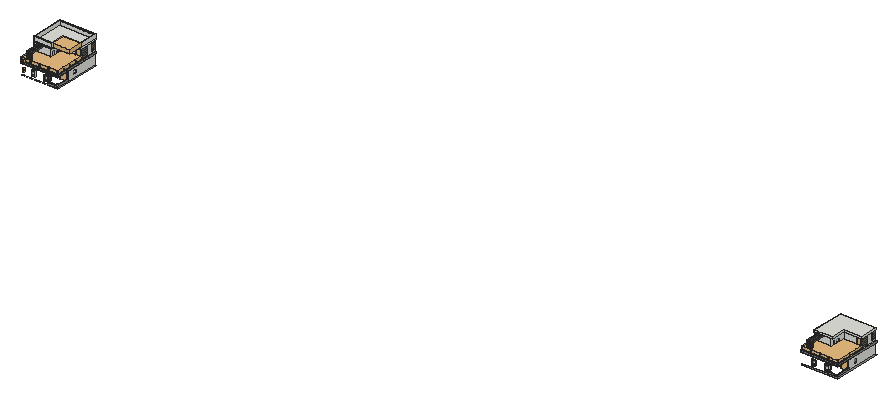
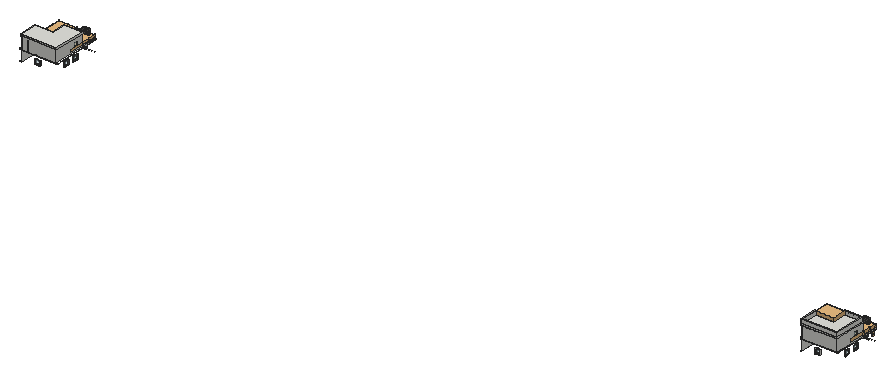
# SketchUp Ruby script. Lengths in inches.
U = 1.inch
M = Sketchup.active_model
def pt(a) = Geom::Point3d.new(a.map { |v| v * U })
def face(e, loops, mat)
  f = e.add_face(loops[0].map { |a| pt(a) })
  loops[1..].each { |l| e.add_face(l.map { |a| pt(a) }).erase! }
  f.material = f.back_material = mat if mat
  f
end
# faces: each face lists its corners as indices into pts; further lists are holes
def faces(e, pts, list, mat = nil) = list.each { |f| face(e, (f[0].is_a?(Array) ? f : [f]).map { |l| l.map { |i| pts[i] } }, mat) }
# xy, xz, yz: faces in a plane at the given z, y or x. An outline is a flat list of corners, or four numbers for a rectangle; further outlines are holes
def ring(l) = l.size == 4 ? [[l[0], l[1]], [l[2], l[1]], [l[2], l[3]], [l[0], l[3]]] : l.each_slice(2).to_a
def flat(e, list, mat, &to3) = list.each { |f| face(e, (f[0].is_a?(Array) ? f : [f]).map { |l| ring(l).map { |u, v| to3.(u, v) } }, mat) }
def xy(e, z, list, mat = nil) = flat(e, list, mat) { |x, y| [x, y, z] }
def xz(e, y, list, mat = nil) = flat(e, list, mat) { |x, z| [x, y, z] }
def yz(e, x, list, mat = nil) = flat(e, list, mat) { |y, z| [x, y, z] }
def lines(e, pts, list) = list.each { |a, b| e.add_line(pt(pts[a]), pt(pts[b])) }
# prism: a flat outline (further loops are holes) pulled along v
def prism(e, loops, v, mat = nil)
  f = face(e, loops, mat); d = Geom::Vector3d.new(v.map { |x| x * U })
  f.pushpull(f.normal.samedirection?(d) ? d.length : -d.length)
end
def box(e, o, s, mat = nil) = prism(e, [[o, [o[0] + s[0], o[1], o[2]], [o[0] + s[0], o[1] + s[1], o[2]], [o[0], o[1] + s[1], o[2]]]], [0, 0, s[2]], mat)
def at(x, y, z, deg = 0) = Geom::Transformation.translation(pt([x, y, z])) * Geom::Transformation.rotation(ORIGIN, Z_AXIS, deg.degrees)
def axes(o, x, y, z) = Geom::Transformation.new([*x, 0, *y, 0, *z, 0, *pt(o).to_a, 1])
def part(name) = M.definitions.add(name)
# library, detail: a bought-in or finely detailed component or shape, given as its bounding box
def library(name, o, s) = part(name).tap { |d| box(d.entities, o, s) }
def detail(e, o, s) = box(e.add_group.entities, o, s)
def put(e, d, t, mat = nil) = e.add_instance(d, t).tap { |i| i.material = mat if mat }
def group(e, t, mat = nil) = e.add_group.tap { |g| g.transformation = t; g.material = mat if mat }.entities
root = M.entities
M.materials.add("Stone C 250cm").color = [107, 104, 102]
M.materials.add("Stone G 100cm").color = [112, 105, 93]
M.materials.add("T8500 Silicone plaster D1 27.81cm").color = [255, 255, 255]
M.materials.add("Wall Paint Bumpy 01 Gray 100cm").color = [135, 135, 135]
M.materials.add("Wood 021 27.52cm").color = [255, 255, 255]
M.materials.add("[Color M06]").color = [86, 86, 86]
M.materials.add("[Translucent Glass Gray]1").color = [128, 128, 128]
M.materials["[Translucent Glass Gray]1"].alpha = 0.5
M.materials.add("[Translucent Glass Safety]").color = [204, 235, 244]
M.materials["[Translucent Glass Safety]"].alpha = 0.5
M.materials.add("[Translucent_Glass_Gray]").color = [128, 128, 128]
M.materials["[Translucent_Glass_Gray]"].alpha = 0.5
c1 = library("Window 46-47",[-61.02,-2.17,0],[122.04,4.34,74.02])
c2 = library("Potted Plant 50-23",[-3.4,-3.5,0],[6.8,7,9.93])
c3 = part("Group\#3")
xy(c3.entities,0,[[0,0,0.83,48],[0.83,0,2.5625,48]])
xy(c3.entities,3,[[0,3,0.67,45],[1.8,3,2.5625,45]])
xy(c3.entities,4.625,[[0.67,4.625,1.8,43.375]])
xy(c3.entities,43.375,[[0.67,4.625,1.8,43.375]])
xy(c3.entities,45,[[0,3,0.67,45],[1.8,3,2.5625,45]])
xy(c3.entities,48,[[0,0,0.83,48],[0.83,0,2.5625,48]])
xz(c3.entities,0,[[0,0,0.83,48],[0.83,0,2.5625,48]])
xz(c3.entities,3,[[0,3,0.67,45],[1.8,3,2.5625,45]])
xz(c3.entities,4.625,[[0.67,4.625,1.8,43.375]])
xz(c3.entities,43.375,[[0.67,4.625,1.8,43.375]])
xz(c3.entities,45,[[0,3,0.67,45],[1.8,3,2.5625,45]])
xz(c3.entities,48,[[0,0,0.83,48],[0.83,0,2.5625,48]])
yz(c3.entities,0,[[[0,0,48,48],[3,3,45,45]]])
yz(c3.entities,0.67,[[[3,3,45,45],[4.625,4.625,43.375,43.375]]])
yz(c3.entities,1.8,[[[3,3,45,45],[4.625,4.625,43.375,43.375]]])
yz(c3.entities,2.5625,[[[0,0,48,48],[3,3,45,45]]])
p = [[1.33,43.375,43.05],[1.33,43.375,4.66],[1.23,4.625,4.66],[1.23,4.625,43.05]]
faces(c3.entities,p,[[0,1,2,3]],"[Translucent Glass Safety]")
c4 = library("Spot Light",[-5.1,-5.1,-11.05],[10.2,10.2,11.05])
c5 = library("Lamp Wall Outdoor 94-02",[-1.89,-4.65,-3.17],[3.78,4.65,6.35])
c6 = part("Group\#7")
p = [[0,43.31,5.11],[2.95,43.31,0],[2.95,0,0],[0,0,5.11]]
faces(c6.entities,p,[[0,1,2,3]],"[Translucent_Glass_Gray]")
c7 = part("Vwntilation window")
put(c7.entities,c6,at(43.48,1.97,32.29))
put(c7.entities,c6,at(43.48,1.97,26.38))
put(c7.entities,c6,at(43.48,1.97,20.48))
put(c7.entities,c6,at(43.48,1.97,14.57))
put(c7.entities,c6,at(43.48,1.97,8.67))
put(c7.entities,c6,at(43.48,1.97,2.76))
g1 = group(c7.entities,at(43.48,0,0))
prism(g1,[[[1.97,47.24,39.37],[1.97,0,39.37],[1.97,0,0],[1.97,47.24,0]],[[1.97,45.28,1.97],[1.97,1.97,1.97],[1.97,1.97,37.4],[1.97,45.28,37.4]]],[-1.97,0,0])
c8 = library("Sphere Light\#7",[-3,-3,-3],[6,6,6])
c9 = library("Sphere Light\#6",[-3,-3,-3],[6,6,6])
c10 = library("Sphere Light\#5",[-3,-3,-3],[6,6,6])
c11 = library("Sphere Light\#8",[-3,-3,-3],[6,6,6])
c12 = library("Door 243 065",[-19.36,-2.49,0],[38.72,4.98,81.96])
c13 = part("Post and beam")
xy(c13.entities,-97.98,[[0,-127.9375,5.5,-124.375]])
xy(c13.entities,0,[[0,-124.375,5.5,0]])
xy(c13.entities,5.4375,[[0,-127.9375,5.5,0]],"Stone C 250cm")
xz(c13.entities,-127.9375,[[0,-97.98,5.5,5.4375]],"Stone C 250cm")
xz(c13.entities,-124.375,[[0,-97.98,5.5,0]])
xz(c13.entities,0,[[0,0,5.5,5.4375]])
yz(c13.entities,0,[[-127.9375,-97.98,-127.9375,5.4375,0,5.4375,0,0,-124.375,0,-124.375,-97.98]],"Stone C 250cm")
yz(c13.entities,5.5,[[-127.9375,-97.98,-124.375,-97.98,-124.375,0,0,0,0,5.4375,-127.9375,5.4375]],"Stone C 250cm")
c14 = part("Group\#6")
xy(c14.entities,0,[[162,13.5,171,46.5],[110.84,153,146.84,162],[298.5,219,331.5,223.5]])
xy(c14.entities,36,[[0,57,9,105],[162,57,171,105]])
xy(c14.entities,84,[[162,13.5,171,46.5],[0,57,9,105],[162,57,171,105],[110.84,153,146.84,162],[298.5,219,331.5,223.5]])
xy(c14.entities,120,[[[0,0,171,0,171,153,351,153,351,328.5,0,328.5],[9,162,9,319.5,342,319.5,342,223.5,294,223.5,294,319.5,289.5,319.5,289.5,219,342,219,342,162],[9,9,162,153]]])
xz(c14.entities,0,[[0,0,171,120]])
xz(c14.entities,9,[[9,0,162,120]])
xz(c14.entities,13.5,[[162,0,171,84]])
xz(c14.entities,46.5,[[162,0,171,84]])
xz(c14.entities,57,[[0,36,9,84],[162,36,171,84]])
xz(c14.entities,105,[[0,36,9,84],[162,36,171,84]])
xz(c14.entities,153,[[9,0,110.84,0,110.84,84,146.84,84,146.84,0,162,0,162,120,9,120],[171,0,351,120]])
xz(c14.entities,162,[[9,0,9,120,342,120,342,0,146.84,0,146.84,84,110.84,84,110.84,0]])
xz(c14.entities,219,[[289.5,0,298.5,0,298.5,84,331.5,84,331.5,0,342,0,342,120,289.5,120]])
xz(c14.entities,223.5,[[294,0,294,120,342,120,342,0,331.5,0,331.5,84,298.5,84,298.5,0]])
xz(c14.entities,319.5,[[9,0,289.5,120],[289.5,0,294,120],[294,0,342,120]])
xz(c14.entities,328.5,[[0,0,351,120]])
yz(c14.entities,0,[[[0,0,328.5,120],[57,36,105,84]]])
yz(c14.entities,9,[[[9,0,153,120],[57,36,105,84]],[162,0,319.5,120]])
yz(c14.entities,110.84,[[153,0,162,84]])
yz(c14.entities,146.84,[[153,0,162,84]])
yz(c14.entities,162,[[[9,0,9,120,153,120,153,0,46.5,0,46.5,84,13.5,84,13.5,0],[57,36,105,84]]])
yz(c14.entities,171,[[[0,0,13.5,0,13.5,84,46.5,84,46.5,0,153,0,153,120,0,120],[57,36,105,84]]])
yz(c14.entities,289.5,[[219,0,319.5,120]])
yz(c14.entities,294,[[223.5,0,319.5,120]])
yz(c14.entities,298.5,[[219,0,223.5,84]])
yz(c14.entities,331.5,[[219,0,223.5,84]])
yz(c14.entities,342,[[162,0,219,120],[223.5,0,319.5,120]])
yz(c14.entities,351,[[153,0,328.5,120]])
c15 = part("Group\#14")
xy(c15.entities,0,[[0,0,2.375,70.51]])
xy(c15.entities,0.3125,[[1.875,0,2.375,70.51]])
xy(c15.entities,0.63,[[1.875,0,2.375,70.51]])
xy(c15.entities,17.3,[[1.875,0,2.375,70.51]])
xy(c15.entities,17.62,[[1.875,0,2.375,70.51]])
xy(c15.entities,34.29,[[1.875,0,2.375,70.51]])
xy(c15.entities,34.61,[[1.875,0,2.375,70.51]])
xy(c15.entities,51.28,[[1.875,0,2.375,70.51]])
xy(c15.entities,51.6,[[1.875,0,2.375,70.51]])
xy(c15.entities,68.28,[[1.875,0,2.375,70.51]])
xy(c15.entities,68.59,[[1.875,0,2.375,70.51]])
xy(c15.entities,85.27,[[1.875,0,2.375,70.51]])
xy(c15.entities,85.58,[[1.875,0,2.375,70.51]],"Stone G 100cm")
xy(c15.entities,102.26,[[1.875,0,2.375,70.51]])
xy(c15.entities,102.57,[[1.875,0,2.375,70.51]])
xy(c15.entities,119.25,[[1.875,0,2.375,70.51]])
xy(c15.entities,119.5625,[[1.875,0,2.375,70.51]],"Stone G 100cm")
xy(c15.entities,120,[[0,0,2.375,70.51]])
xz(c15.entities,0,[[0,0,2.375,0.3125],[0,0.3125,1.875,0.63],[0,17.3,1.875,17.62],[0,34.29,1.875,34.61],[0,51.28,1.875,51.6],
  [0,68.28,1.875,68.59],[0,85.27,1.875,85.58],[0,102.26,1.875,102.57],[0,119.25,1.875,119.5625],[0,119.5625,2.375,120]])
xz(c15.entities,0,[[0,0.63,2.375,17.3],[0,17.62,2.375,34.29],[0,34.61,2.375,51.28],[0,51.6,2.375,68.28],[0,68.59,2.375,85.27],
  [0,85.58,2.375,102.26],[0,102.57,2.375,119.25]],"Stone G 100cm")
xz(c15.entities,70.51,[[0,102.26,1.875,102.57]])
xz(c15.entities,70.51,[[0,0,2.375,0.3125],[0,0.3125,1.875,0.63],[0,0.63,2.375,17.3],[0,17.3,1.875,17.62],[0,17.62,2.375,34.29],
  [0,34.29,1.875,34.61],[0,34.61,2.375,51.28],[0,51.28,1.875,51.6],[0,51.6,2.375,68.28],[0,68.28,1.875,68.59],
  [0,68.59,2.375,85.27],[0,85.27,1.875,85.58],[0,85.58,2.375,102.26],[0,102.57,2.375,119.25],[0,119.25,1.875,119.5625],
  [0,119.5625,2.375,120]],"Stone G 100cm")
yz(c15.entities,0,[[0,0,70.51,120]])
yz(c15.entities,1.875,[[0,119.25,70.51,119.5625]])
yz(c15.entities,1.875,[[0,0.3125,70.51,0.63],[0,17.3,70.51,17.62],[0,34.29,70.51,34.61],[0,51.28,70.51,51.6],[0,68.28,70.51,68.59],
  [0,85.27,70.51,85.58],[0,102.26,70.51,102.57]],"Stone G 100cm")
yz(c15.entities,2.375,[[0,0,70.51,0.3125],[0,0.63,70.51,17.3],[0,17.62,70.51,34.29],[0,34.61,70.51,51.28],[0,51.6,70.51,68.28],
  [0,68.59,70.51,85.27],[0,85.58,70.51,102.26],[0,102.57,70.51,119.25],[0,119.5625,70.51,120]],"Stone G 100cm")
c16 = library("Group\#16",[0,0,0],[44.53,1,120])
c17 = library("Potted Plant 02",[-16.98,-19.78,0],[30.04,38.68,37.52])
c18 = library("Group61\#1",[7976.64,457.72,288.35],[367.58,308.29,25.19])
c19 = library("Ploe",[7975.85,611.43,276.75],[3.15,3.15,37.57])
c20 = part("Group60\#1")
put(c20.entities,c19,at(0,0,0))
put(c20.entities,c19,at(0,-77.25,0))
put(c20.entities,c19,at(0,-154.5,0))
put(c20.entities,c19,at(91.5,-154.5,0))
put(c20.entities,c19,at(183,-154.5,0))
put(c20.entities,c19,at(274.5,-154.5,0))
put(c20.entities,c19,at(366,-154.5,0))
put(c20.entities,c19,at(366,-77.625,0))
put(c20.entities,c19,at(366,-0.75,0))
put(c20.entities,c19,at(366,76.125,0))
put(c20.entities,c19,at(366,153,0))
c21 = part("Group\#11")
put(c21.entities,c18,at(-7975.85,-456.93,-276.75))
put(c21.entities,c20,at(-7975.85,-456.93,-276.75))
c22 = part("Group\#15")
prism(c22.entities,[[[0,0,109.9375],[0,0,0],[2.375,0,0],[2.375,0,0.5],[0.75,0,0.5],[0.75,0,1.5],[2.375,0,1.5],[2.375,0,21.99],[0.75,0,21.99],[0.75,0,22.99],[2.375,0,22.99],[2.375,0,43.48],[0.75,0,43.48],[0.75,0,44.48],[2.375,0,44.48],[2.375,0,64.96],[0.75,0,64.96],[0.75,0,65.96],[2.375,0,65.96],[2.375,0,86.45],[0.75,0,86.45],[0.75,0,87.45],[2.375,0,87.45],[2.375,0,107.9375],[0.75,0,107.9375],[0.75,0,108.9375],[2.375,0,108.9375],[2.375,0,109.9375]]],[0,39.5,0],"Stone G 100cm")
c23 = library("Sphere Light\#4",[-2,-2,-2],[4,4,4])
c24 = library("Sphere Light",[-2,-2,-2],[4,4,4])
c25 = library("Sphere Light\#3",[-2,-2,-2],[4,4,4])
c26 = library("Sphere Light\#2",[-2,-2,-2],[4,4,4])
c27 = library("Sphere Light\#1",[-2,-2,-2],[4,4,4])
c28 = library("Group\#21",[0,0,0],[182.86,140.18,36.98])
xy(root,144.75,[[686.23,450.625,758.23,459.625],[8453.94,661.9,8525.94,670.9]])
xy(root,152.75,[[420.73,290.125,786.73,290.125,786.73,779.125,771.73,779.125,771.73,302.125,475.97,302.125,475.97,293.5625,420.73,293.5625],[8188.44,501.4,8554.44,501.4,8554.44,990.4,8539.44,990.4,8539.44,513.4,8243.6875,513.4,8243.6875,504.84,8188.44,504.84]],"Wall Paint Bumpy 01 Gray 100cm")
xy(root,169.375,[[681.73,302.125,681.73,311.125,762.73,311.125,762.73,450.625,771.73,450.625,771.73,302.125],[8449.44,513.4,8449.44,522.4,8530.44,522.4,8530.44,661.9,8539.44,661.9,8539.44,513.4]])
xy(root,170.375,[[681.73,302.125,771.73,302.125,771.73,450.625,762.73,450.625,762.73,311.125,681.73,311.125],[8449.44,513.4,8539.44,513.4,8539.44,661.9,8530.44,661.9,8530.44,522.4,8449.44,522.4]],"T8500 Silicone plaster D1 27.81cm")
xy(root,176.75,[[512.01,302.125,548.01,311.125],[641.23,302.125,681.73,302.125,681.73,335.125,681.13,335.125,681.13,304.97,641.23,304.97],[641.23,306.1,680.01,306.1,680.01,335.125,679.48,335.125,679.48,306.625,641.23,306.625],[641.23,306.625,679.48,306.625,679.48,335.125,677.23,335.125,677.23,311.125,641.23,311.125],[420.73,507.625,429.73,555.625],
  [762.73,507.625,771.73,555.625],[8279.73,513.4,8315.73,522.4],[8408.94,513.4,8449.44,513.4,8449.44,546.4,8448.85,546.4,8448.85,516.25,8408.94,516.25],[8408.94,517.375,8447.72,517.375,8447.72,546.4,8447.19,546.4,8447.19,517.9,8408.94,517.9],[8408.94,517.9,8447.19,517.9,8447.19,546.4,8444.94,546.4,8444.94,522.4,8408.94,522.4],
  [420.73,618.96,429.73,666.96],[8188.44,718.9,8197.44,766.9],[8530.44,718.9,8539.44,766.9],[590.04,770.125,638.04,779.125],[8188.44,830.24,8197.44,878.24],
  [8357.75,981.4,8405.75,990.4]])
xy(root,178.125,[[642.6,304.97,681.13,304.97,681.13,333.75,680.88,333.75,680.88,305.22,642.6,305.22],[642.6,305.79,680.32,305.79,680.32,333.75,680.01,333.75,680.01,306.1,642.6,306.1],[8410.32,516.25,8448.85,516.25,8448.85,545.03,8448.6,545.03,8448.6,516.5,8410.32,516.5],[8410.32,517.07,8448.03,517.07,8448.03,545.03,8447.72,545.03,8447.72,517.375,8410.32,517.375]])
xy(root,178.8125,[[643.29,305.22,680.88,305.22,680.88,333.0625,680.32,333.0625,680.32,305.79,643.29,305.79],[8411.01,516.5,8448.6,516.5,8448.6,544.34,8448.03,544.34,8448.03,517.07,8411.01,517.07]])
xy(root,222.6875,[[643.29,305.22,643.29,305.79,680.32,305.79,680.32,333.0625,680.88,333.0625,680.88,305.22],[8411.01,516.5,8411.01,517.07,8448.03,517.07,8448.03,544.34,8448.6,544.34,8448.6,516.5]])
xy(root,223.375,[[642.6,304.97,642.6,305.22,680.88,305.22,680.88,333.75,681.13,333.75,681.13,304.97],[642.6,305.79,642.6,306.1,680.01,306.1,680.01,333.75,680.32,333.75,680.32,305.79],[8410.32,516.25,8410.32,516.5,8448.6,516.5,8448.6,545.03,8448.85,545.03,8448.85,516.25],[8410.32,517.07,8410.32,517.375,8447.72,517.375,8447.72,545.03,8448.03,545.03,8448.03,517.07]])
xy(root,224.75,[[512.01,302.125,548.01,311.125],[641.23,302.125,641.23,304.97,681.13,304.97,681.13,335.125,681.73,335.125,681.73,302.125],[641.23,306.1,641.23,306.625,679.48,306.625,679.48,335.125,680.01,335.125,680.01,306.1],[641.23,306.625,641.23,311.125,677.23,311.125,677.23,335.125,679.48,335.125,679.48,306.625],[452.23,360.625,485.23,365.125],
  [633.73,455.125,672.73,459.625],[420.73,507.625,429.73,555.625],[762.73,507.625,771.73,555.625],[8279.73,513.4,8315.73,522.4],[8408.94,513.4,8408.94,516.25,8448.85,516.25,8448.85,546.4,8449.44,546.4,8449.44,513.4],
  [8408.94,517.375,8408.94,517.9,8447.19,517.9,8447.19,546.4,8447.72,546.4,8447.72,517.375],[8408.94,517.9,8408.94,522.4,8444.94,522.4,8444.94,546.4,8447.19,546.4,8447.19,517.9],[8219.94,571.9,8252.94,576.4],[594.73,603.625,633.73,608.125],[420.73,618.96,429.73,666.96],
  [8401.44,666.4,8440.44,670.9],[671.23,680.125,704.23,684.625],[8188.44,718.9,8197.44,766.9],[8530.44,718.9,8539.44,766.9],[590.04,770.125,638.04,779.125],
  [8362.44,814.9,8401.44,819.4],[8188.44,830.24,8197.44,878.24],[8438.94,891.4,8471.94,895.9],[8357.75,981.4,8405.75,990.4]])
xy(root,230.75,[[420.73,387.69,429.73,411.65],[8188.44,598.97,8197.44,622.93],[762.73,691.19,771.73,715.15],[8530.44,902.47,8539.44,926.43]])
xy(root,240.75,[[686.23,450.625,758.23,459.625],[8453.94,661.9,8525.94,670.9]])
xy(root,248.75,[[420.73,387.69,429.73,411.65],[8188.44,598.97,8197.44,622.93],[645.73,644.125,650.23,680.125],[762.73,691.19,771.73,715.15],[8413.44,855.4,8417.94,891.4],
  [8530.44,902.47,8539.44,926.43]])
xy(root,259.75,[[681.73,325.25,681.73,450.25,733.17,450.25,726.6,325.25],[726.6,325.25,733.17,450.25,771.48,450.25,771.48,325.25]])
xy(root,260.75,[[420.73,302.125,681.73,302.125,681.73,450.625,762.73,450.625,762.73,459.625,429.73,459.625,429.73,455.125,489.73,455.125,489.73,365.125,429.73,365.125,429.73,360.625,494.23,360.625,494.23,455.125,677.23,455.125,677.23,311.125,429.73,311.125,429.73,770.125,762.73,770.125,762.73,450.625,771.73,450.625,771.73,779.125,420.73,779.125],[8188.44,513.4,8449.44,513.4,8449.44,661.9,8530.44,661.9,8530.44,670.9,8197.44,670.9,8197.44,666.4,8257.44,666.4,8257.44,576.4,8197.44,576.4,8197.44,571.9,8261.94,571.9,8261.94,666.4,8444.94,666.4,8444.94,522.4,8197.44,522.4,8197.44,981.4,8530.44,981.4,8530.44,661.9,8539.44,661.9,8539.44,990.4,8188.44,990.4],[429.73,603.625,762.73,603.625,762.73,608.125,650.23,608.125,650.23,680.125,762.73,680.125,762.73,684.625,650.23,684.625,650.23,770.125,645.73,770.125,645.73,608.125,429.73,608.125],[8197.44,814.9,8530.44,814.9,8530.44,819.4,8417.94,819.4,8417.94,891.4,8530.44,891.4,8530.44,895.9,8417.94,895.9,8417.94,981.4,8413.44,981.4,8413.44,819.4,8197.44,819.4]])
xy(root,260.75,[[681.73,325.25,771.48,450.25]],"Wood 021 27.52cm")
xy(root,264.75,[[408.73,290.125,408.73,450.625,420.73,450.625,420.73,302.125,774.73,302.125,774.73,775.5,771.73,775.5,771.73,779.125,786.73,779.125,786.73,290.125],[8176.44,501.4,8176.44,661.9,8188.44,661.9,8188.44,513.4,8542.44,513.4,8542.44,986.78,8539.44,986.78,8539.44,990.4,8554.44,990.4,8554.44,501.4]])
xy(root,276.75,[[408.73,290.125,786.73,290.125,786.73,779.125,771.73,779.125,771.73,775.5,774.73,775.5,774.73,302.125,420.73,302.125,420.73,450.625,408.73,450.625],[8176.44,501.4,8554.44,501.4,8554.44,990.4,8539.44,990.4,8539.44,986.78,8542.44,986.78,8542.44,513.4,8188.44,513.4,8188.44,661.9,8176.44,661.9]])
xy(root,401.1875,[[432.73,457.625,594.73,457.625,594.73,600.625,774.73,600.625,774.73,767.125,432.73,767.125],[594.73,457.625,606.73,457.625,606.73,588.89,774.73,588.89,774.73,588.625,786.73,588.625,786.73,595.11,774.73,595.11,774.73,600.625,594.73,600.625]])
xy(root,438.17,[[420.73,445.625,606.73,457.625],[420.73,457.625,432.73,457.625,432.73,767.125,774.73,767.125,774.73,595.11,786.73,595.11,786.73,779.125,420.73,779.125]])
xz(root,290.125,[[408.73,264.75,786.73,276.75]],"Wall Paint Bumpy 01 Gray 100cm")
xz(root,302.125,[[420.73,264.75,774.73,276.75]])
xz(root,302.125,[[681.73,169.375,771.73,170.375]],"T8500 Silicone plaster D1 27.81cm")
xz(root,302.125,[[681.73,152.75,771.73,169.375]],"Wall Paint Bumpy 01 Gray 100cm")
xz(root,304.97,[[641.23,176.75,681.13,176.75,681.13,178.125,642.6,178.125,642.6,223.375,681.13,223.375,681.13,224.75,641.23,224.75]])
xz(root,305.22,[[642.6,178.125,680.88,178.125,680.88,178.8125,643.29,178.8125,643.29,222.6875,680.88,222.6875,680.88,223.375,642.6,223.375]])
xz(root,305.22,[[643.29,178.8125,680.88,222.6875]],"[Translucent Glass Gray]1")
xz(root,305.79,[[642.6,178.125,642.6,223.375,680.32,223.375,680.32,222.6875,643.29,222.6875,643.29,178.8125,680.32,178.8125,680.32,178.125]])
xz(root,306.1,[[641.23,176.75,641.23,224.75,680.01,224.75,680.01,223.375,642.6,223.375,642.6,178.125,680.01,178.125,680.01,176.75]])
xz(root,311.125,[[681.73,169.375,762.73,170.375]])
xz(root,325.25,[[681.73,259.75,771.48,260.75]],"Wood 021 27.52cm")
xz(root,333.0625,[[680.32,178.8125,680.88,222.6875]])
xz(root,333.75,[[680.01,178.125,680.32,223.375],[680.88,178.125,681.13,223.375]])
xz(root,335.125,[[677.23,176.75,679.48,224.75],[679.48,176.75,680.01,224.75],[681.13,176.75,681.73,224.75]])
xz(root,387.69,[[420.73,230.75,429.73,248.75]])
xz(root,411.65,[[420.73,230.75,429.73,248.75]])
xz(root,445.625,[[420.73,401.1875,606.73,438.17]])
xz(root,450.25,[[681.73,259.75,771.48,260.75]])
xz(root,450.625,[[762.73,169.375,771.73,170.375],[762.73,170.375,771.73,260.75],[408.73,264.75,420.73,276.75]])
xz(root,457.625,[[432.73,401.1875,594.73,438.17],[594.73,401.1875,606.73,438.17]])
xz(root,501.4,[[8176.44,264.75,8554.44,276.75]],"Wall Paint Bumpy 01 Gray 100cm")
xz(root,507.625,[[420.73,176.75,429.73,224.75],[762.73,176.75,771.73,224.75]])
xz(root,513.4,[[8188.44,264.75,8542.44,276.75]])
xz(root,513.4,[[8449.44,169.375,8539.44,170.375]],"T8500 Silicone plaster D1 27.81cm")
xz(root,513.4,[[8449.44,152.75,8539.44,169.375]],"Wall Paint Bumpy 01 Gray 100cm")
xz(root,516.25,[[8408.94,176.75,8448.85,176.75,8448.85,178.125,8410.32,178.125,8410.32,223.375,8448.85,223.375,8448.85,224.75,8408.94,224.75]])
xz(root,516.5,[[8410.32,178.125,8448.6,178.125,8448.6,178.8125,8411.01,178.8125,8411.01,222.6875,8448.6,222.6875,8448.6,223.375,8410.32,223.375]])
xz(root,516.5,[[8411.01,178.8125,8448.6,222.6875]],"[Translucent Glass Gray]1")
xz(root,517.07,[[8410.32,178.125,8410.32,223.375,8448.03,223.375,8448.03,222.6875,8411.01,222.6875,8411.01,178.8125,8448.03,178.8125,8448.03,178.125]])
xz(root,517.375,[[8408.94,176.75,8408.94,224.75,8447.72,224.75,8447.72,223.375,8410.32,223.375,8410.32,178.125,8447.72,178.125,8447.72,176.75]])
xz(root,522.4,[[8449.44,169.375,8530.44,170.375]])
xz(root,544.34,[[8448.03,178.8125,8448.6,222.6875]])
xz(root,545.03,[[8447.72,178.125,8448.03,223.375],[8448.6,178.125,8448.85,223.375]])
xz(root,546.4,[[8444.94,176.75,8447.19,224.75],[8447.19,176.75,8447.72,224.75],[8448.85,176.75,8449.44,224.75]])
xz(root,555.625,[[420.73,176.75,429.73,224.75],[762.73,176.75,771.73,224.75]])
xz(root,595.11,[[774.73,401.1875,786.73,438.17]])
xz(root,598.97,[[8188.44,230.75,8197.44,248.75]])
xz(root,618.96,[[420.73,176.75,429.73,224.75]])
xz(root,622.93,[[8188.44,230.75,8197.44,248.75]])
xz(root,661.9,[[8530.44,169.375,8539.44,170.375],[8530.44,170.375,8539.44,260.75],[8176.44,264.75,8188.44,276.75]])
xz(root,666.96,[[420.73,176.75,429.73,224.75]])
xz(root,691.19,[[762.73,230.75,771.73,248.75]])
xz(root,715.15,[[762.73,230.75,771.73,248.75]])
xz(root,718.9,[[8188.44,176.75,8197.44,224.75],[8530.44,176.75,8539.44,224.75]])
xz(root,766.9,[[8188.44,176.75,8197.44,224.75],[8530.44,176.75,8539.44,224.75]])
xz(root,767.125,[[432.73,401.1875,774.73,438.17]])
xz(root,775.5,[[771.73,264.75,774.73,276.75]])
xz(root,779.125,[[771.73,264.75,786.73,276.75],[420.73,401.1875,786.73,438.17]])
xz(root,830.24,[[8188.44,176.75,8197.44,224.75]])
xz(root,878.24,[[8188.44,176.75,8197.44,224.75]])
xz(root,902.47,[[8530.44,230.75,8539.44,248.75]])
xz(root,926.43,[[8530.44,230.75,8539.44,248.75]])
xz(root,986.78,[[8539.44,264.75,8542.44,276.75]])
xz(root,990.4,[[8539.44,264.75,8554.44,276.75]])
yz(root,408.73,[[290.125,264.75,450.625,276.75]])
yz(root,420.73,[[302.125,264.75,450.625,276.75],[445.625,401.1875,457.625,438.17],[457.625,401.1875,779.125,438.17]])
yz(root,432.73,[[457.625,401.1875,767.125,438.17]])
yz(root,512.01,[[302.125,176.75,311.125,224.75]])
yz(root,548.01,[[302.125,176.75,311.125,224.75]])
yz(root,590.04,[[770.125,176.75,779.125,224.75]])
yz(root,606.73,[[445.625,401.1875,457.625,438.17]])
yz(root,638.04,[[770.125,176.75,779.125,224.75]])
yz(root,641.23,[[302.125,176.75,304.97,224.75],[306.1,176.75,306.625,224.75],[306.625,176.75,311.125,224.75]])
yz(root,642.6,[[304.97,178.125,305.22,223.375],[305.79,178.125,306.1,223.375]])
yz(root,643.29,[[305.22,178.8125,305.79,222.6875]])
yz(root,680.01,[[306.1,176.75,306.1,178.125,333.75,178.125,333.75,223.375,306.1,223.375,306.1,224.75,335.125,224.75,335.125,176.75]])
yz(root,680.32,[[305.79,178.125,305.79,178.8125,333.0625,178.8125,333.0625,222.6875,305.79,222.6875,305.79,223.375,333.75,223.375,333.75,178.125]])
yz(root,680.88,[[305.22,178.125,333.75,178.125,333.75,223.375,305.22,223.375,305.22,222.6875,333.0625,222.6875,333.0625,178.8125,305.22,178.8125]])
yz(root,680.88,[[305.22,178.8125,333.0625,222.6875]],"[Translucent Glass Gray]1")
yz(root,681.13,[[304.97,176.75,335.125,176.75,335.125,224.75,304.97,224.75,304.97,223.375,333.75,223.375,333.75,178.125,304.97,178.125]])
yz(root,681.73,[[302.125,169.375,311.125,170.375],[325.25,259.75,450.25,260.75]])
yz(root,686.23,[[450.625,144.75,459.625,240.75]])
yz(root,758.23,[[450.625,144.75,459.625,240.75]])
yz(root,762.73,[[311.125,169.375,450.625,170.375]])
yz(root,771.48,[[325.25,259.75,450.25,260.75]],"Wood 021 27.52cm")
yz(root,771.73,[[[450.625,152.75,779.125,260.75],[507.625,176.75,555.625,224.75],[691.19,230.75,715.15,248.75]],[775.5,264.75,779.125,276.75]])
yz(root,771.73,[[302.125,169.375,450.625,170.375]],"T8500 Silicone plaster D1 27.81cm")
yz(root,771.73,[[302.125,152.75,450.625,169.375]],"Wall Paint Bumpy 01 Gray 100cm")
yz(root,774.73,[[302.125,264.75,775.5,276.75],[595.11,401.1875,767.125,438.17]])
yz(root,786.73,[[595.11,401.1875,779.125,438.17]])
yz(root,786.73,[[290.125,264.75,779.125,276.75]],"Wall Paint Bumpy 01 Gray 100cm")
yz(root,8176.44,[[501.4,264.75,661.9,276.75]])
yz(root,8188.44,[[513.4,264.75,661.9,276.75]])
yz(root,8279.73,[[513.4,176.75,522.4,224.75]])
yz(root,8315.73,[[513.4,176.75,522.4,224.75]])
yz(root,8357.75,[[981.4,176.75,990.4,224.75]])
yz(root,8405.75,[[981.4,176.75,990.4,224.75]])
yz(root,8408.94,[[513.4,176.75,516.25,224.75],[517.375,176.75,517.9,224.75],[517.9,176.75,522.4,224.75]])
yz(root,8410.32,[[516.25,178.125,516.5,223.375],[517.07,178.125,517.375,223.375]])
yz(root,8411.01,[[516.5,178.8125,517.07,222.6875]])
yz(root,8447.72,[[517.375,176.75,517.375,178.125,545.03,178.125,545.03,223.375,517.375,223.375,517.375,224.75,546.4,224.75,546.4,176.75]])
yz(root,8448.03,[[517.07,178.125,517.07,178.8125,544.34,178.8125,544.34,222.6875,517.07,222.6875,517.07,223.375,545.03,223.375,545.03,178.125]])
yz(root,8448.6,[[516.5,178.125,545.03,178.125,545.03,223.375,516.5,223.375,516.5,222.6875,544.34,222.6875,544.34,178.8125,516.5,178.8125]])
yz(root,8448.6,[[516.5,178.8125,544.34,222.6875]],"[Translucent Glass Gray]1")
yz(root,8448.85,[[516.25,176.75,546.4,176.75,546.4,224.75,516.25,224.75,516.25,223.375,545.03,223.375,545.03,178.125,516.25,178.125]])
yz(root,8449.44,[[513.4,169.375,522.4,170.375]])
yz(root,8453.94,[[661.9,144.75,670.9,240.75]])
yz(root,8525.94,[[661.9,144.75,670.9,240.75]])
yz(root,8530.44,[[522.4,169.375,661.9,170.375]])
yz(root,8539.44,[[[661.9,152.75,990.4,260.75],[718.9,176.75,766.9,224.75],[902.47,230.75,926.43,248.75]],[986.78,264.75,990.4,276.75]])
yz(root,8539.44,[[513.4,169.375,661.9,170.375]],"T8500 Silicone plaster D1 27.81cm")
yz(root,8539.44,[[513.4,152.75,661.9,169.375]],"Wall Paint Bumpy 01 Gray 100cm")
yz(root,8542.44,[[513.4,264.75,986.78,276.75]])
yz(root,8554.44,[[501.4,264.75,990.4,276.75]],"Wall Paint Bumpy 01 Gray 100cm")
p = [[8410.6,516.5,178.8125],[8410.6,516.5,222.6875],[8411.01,516.51,222.6875],[8448.3,516.78,222.6875],[8448.3,516.78,178.8125],[8411.01,516.51,178.8125],
  [8448.6,516.5,222.6875],[8448.25,544.15,222.6875],[8448.25,544.15,178.8125],[8448.6,516.5,178.8125],[680.59,305.5,222.6875],[680.59,305.5,178.8125],
  [643.29,305.23,178.8125],[642.89,305.22,222.6875],[643.29,305.23,222.6875],[642.89,305.22,178.8125],[680.88,305.22,222.6875],[680.54,332.87,222.6875],
  [680.54,332.87,178.8125],[680.88,305.22,178.8125]]
lines(root,p,[[0,1],[1,2],[3,4],[4,5],[2,3],[5,0],[6,7],[7,8],[8,9],[10,11],[11,12],[13,14],
  [14,10],[15,13],[12,15],[16,17],[18,19],[17,18]])
put(root,c1,axes([722.22,455.03,144.41],[0.59005,0,0],[0,2.0358,0],[0,0,1.30159]))
put(root,c1,axes([8489.9375,666.3125,144.41],[0.59005,0,0],[0,2.0358,0],[0,0,1.30159]))
put(root,c2,at(767.22,442.75,170.375))
put(root,c2,at(769.32,308.68,170.375))
put(root,c2,at(687.2,304.32,170.375))
put(root,c3,axes([548.01,306.625,176.75],[0,1,0],[-0.75,0,0],[0,0,1]),"[Color M06]")
put(root,c3,axes([8315.73,517.9,176.75],[0,1,0],[-0.75,0,0],[0,0,1]),"[Color M06]")
put(root,c3,at(590.04,772.6875,176.75,-90),"[Color M06]")
put(root,c3,at(8357.75,983.97,176.75,-90),"[Color M06]")
put(root,c3,at(764.67,507.625,176.75),"[Color M06]")
put(root,c3,at(8532.38,718.9,176.75),"[Color M06]")
put(root,c3,at(424.4,618.96,176.75),"[Color M06]")
put(root,c3,at(8192.11,830.24,176.75),"[Color M06]")
put(root,c3,at(425.23,507.625,176.75),"[Color M06]")
put(root,c3,at(8192.94,718.9,176.75),"[Color M06]")
put(root,c4,at(442.71,291.26,204.68))
put(root,c5,axes([442.71,293.5625,210.11],[2.22,0,0],[0,1,0],[0,0,1.71]))
put(root,c4,axes([442.99,289,216.64],[1,0,0],[0,-1,0],[0,0,-1]))
put(root,c7,axes([396.02,387.57,230.75],[0.67181,0,0],[0,0.50965,0],[0,0,0.4572]))
put(root,c7,axes([8163.73,598.85,230.75],[0.67181,0,0],[0,0.50965,0],[0,0,0.4572]))
put(root,c7,axes([738.02,691.07,230.75],[0.67181,0,0],[0,0.50965,0],[0,0,0.4572]))
put(root,c7,axes([8505.73,902.35,230.75],[0.67181,0,0],[0,0.50965,0],[0,0,0.4572]))
put(root,c8,at(707.88,426.25,259.75))
put(root,c9,at(752.12,353.38,259.75))
put(root,c10,at(704.05,353.38,259.75))
put(root,c11,at(755.95,426.25,259.75))
g2 = group(root,at(681.73,325.25,259.75))
xy(g2,0,[[0,0,89.75,125]],"Wood 021 27.52cm")
p = [[89.75,0,1],[0,0,1],[89.75,125,1]]
lines(g2,p,[[0,1],[2,0]])
g3 = group(root,at(420.73,303.57,260.75))
box(g3,[-12,-13.45,0],[378,489,4],"T8500 Silicone plaster D1 27.81cm")
g4 = group(root,at(8188.44,514.85,260.75))
box(g4,[-12,-13.45,0],[378,489,4],"T8500 Silicone plaster D1 27.81cm")
put(root,c12,axes([584.81,480.6875,264.64],[0.00001,0.84915,0.00245],[-1,0,0.00289],[0.00296,-0.00296,1.02399]))
put(root,c12,axes([8352.52,691.97,264.64],[0.00001,0.84915,0.00245],[-1,0,0.00289],[0.00296,-0.00296,1.02399]))
put(root,c13,at(471.52,450.625,362.73))
put(root,c13,at(496.05,450.625,362.73))
put(root,c13,at(446.98,450.625,362.73))
put(root,c13,at(459.25,450.625,362.73))
put(root,c13,at(483.78,450.625,362.73))
put(root,c14,at(420.73,450.625,264.75))
put(root,c13,at(8214.7,661.9,362.73))
put(root,c13,at(8226.97,661.9,362.73))
put(root,c13,at(8239.23,661.9,362.73))
put(root,c13,at(8251.5,661.9,362.73))
put(root,c13,at(8263.76,661.9,362.73))
put(root,c14,at(8188.44,661.9,264.75))
put(root,c15,at(771.73,603.625,264.75))
put(root,c16,at(727.2,602.625,264.75))
put(root,c15,at(8539.44,814.9,264.75))
put(root,c16,at(8494.92,813.9,264.75))
put(root,c17,at(758.44,323.04,264.75))
put(root,c17,at(434.73,311.53,264.75))
put(root,c21,at(413.15,294.55,276.75))
put(root,c21,at(8180.87,505.83,276.75))
put(root,c3,at(584.67,507.625,300.75),"[Color M06]")
put(root,c3,at(8352.38,718.9,300.75),"[Color M06]")
put(root,c3,at(425.23,507.625,300.75),"[Color M06]")
put(root,c3,at(8192.94,718.9,300.75),"[Color M06]")
put(root,c22,axes([771.73,739.625,304.49],[1,0,0],[0,1,0],[0,0,0.73]))
put(root,c22,axes([8539.44,950.9,304.49],[1,0,0],[0,1,0],[0,0,0.73]))
put(root,c23,at(778.49,707.44,384.75))
put(root,c24,at(613.09,596.33,384.75))
put(root,c25,at(757.02,596.33,384.75))
put(root,c26,at(699.59,596.33,384.75))
put(root,c27,at(657.57,596.33,384.75))
g5 = group(root,at(420.73,303.57,384.75))
prism(g5,[[[366,475.55,0],[366,285.05,0],[186,285.05,0],[186,142.05,0],[0,142.05,0],[0,475.55,0]]],[0,0,16.4375])
g6 = group(root,at(8188.44,514.85,384.75))
prism(g6,[[[366,475.55,0],[366,285.05,0],[186,285.05,0],[186,142.05,0],[0,142.05,0],[0,475.55,0]]],[0,0,16.4375])
put(root,c28,at(599.55,455.66,401.1875))
